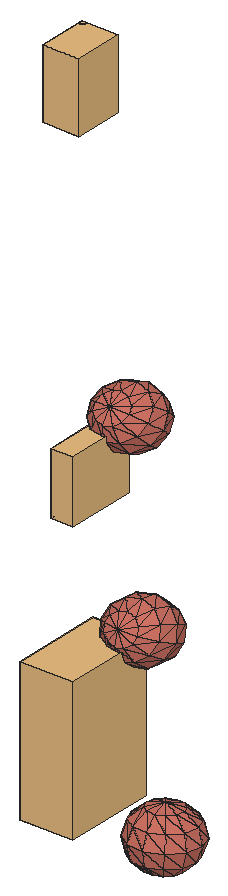
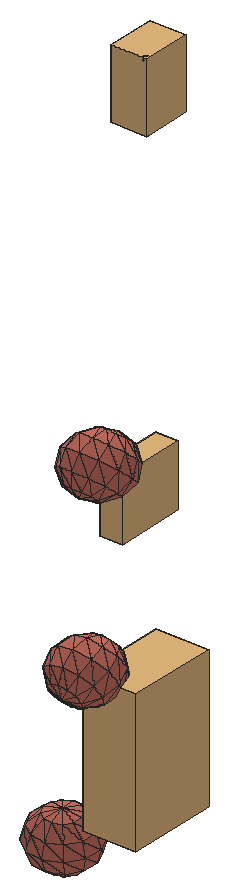
# SketchUp Ruby script. Lengths in inches.
U = 1.inch
M = Sketchup.active_model
def pt(a) = Geom::Point3d.new(a.map { |v| v * U })
def face(e, loops, mat)
  f = e.add_face(loops[0].map { |a| pt(a) })
  loops[1..].each { |l| e.add_face(l.map { |a| pt(a) }).erase! }
  f.material = f.back_material = mat if mat
  f
end
# faces: each face lists its corners as indices into pts; further lists are holes
def faces(e, pts, list, mat = nil) = list.each { |f| face(e, (f[0].is_a?(Array) ? f : [f]).map { |l| l.map { |i| pts[i] } }, mat) }
# xy, xz, yz: faces in a plane at the given z, y or x. An outline is a flat list of corners, or four numbers for a rectangle; further outlines are holes
def ring(l) = l.size == 4 ? [[l[0], l[1]], [l[2], l[1]], [l[2], l[3]], [l[0], l[3]]] : l.each_slice(2).to_a
def flat(e, list, mat, &to3) = list.each { |f| face(e, (f[0].is_a?(Array) ? f : [f]).map { |l| ring(l).map { |u, v| to3.(u, v) } }, mat) }
def xy(e, z, list, mat = nil) = flat(e, list, mat) { |x, y| [x, y, z] }
def xz(e, y, list, mat = nil) = flat(e, list, mat) { |x, z| [x, y, z] }
def yz(e, x, list, mat = nil) = flat(e, list, mat) { |y, z| [x, y, z] }
def lines(e, pts, list) = list.each { |a, b| e.add_line(pt(pts[a]), pt(pts[b])) }
# prism: a flat outline (further loops are holes) pulled along v
def prism(e, loops, v, mat = nil)
  f = face(e, loops, mat); d = Geom::Vector3d.new(v.map { |x| x * U })
  f.pushpull(f.normal.samedirection?(d) ? d.length : -d.length)
end
def box(e, o, s, mat = nil) = prism(e, [[o, [o[0] + s[0], o[1], o[2]], [o[0] + s[0], o[1] + s[1], o[2]], [o[0], o[1] + s[1], o[2]]]], [0, 0, s[2]], mat)
def at(x, y, z, deg = 0) = Geom::Transformation.translation(pt([x, y, z])) * Geom::Transformation.rotation(ORIGIN, Z_AXIS, deg.degrees)
def axes(o, x, y, z) = Geom::Transformation.new([*x, 0, *y, 0, *z, 0, *pt(o).to_a, 1])
def part(name) = M.definitions.add(name)
# library, detail: a bought-in or finely detailed component or shape, given as its bounding box
def library(name, o, s) = part(name).tap { |d| box(d.entities, o, s) }
def detail(e, o, s) = box(e.add_group.entities, o, s)
def put(e, d, t, mat = nil) = e.add_instance(d, t).tap { |i| i.material = mat if mat }
def group(e, t, mat = nil) = e.add_group.tap { |g| g.transformation = t; g.material = mat if mat }.entities
root = M.entities
M.materials.add("green").color = [174, 139, 102]
M.materials.add("vio").color = [206, 114, 100]
c1 = library("3DGeom~25_Defintion",[-351.97,-500,-258.4],[703.94,1000,516.8])
c2 = part("3DGeom~26_Defintion")
p = [[-344.73,487.39,-243.89],[-293.86,494.46,-251.4],[-311.18,491.2,-258.4],[-344.73,487.39,-243.89],[-311.18,491.2,-258.4],[-329.79,488.61,-255.65],
  [-344.73,487.39,-243.89],[-282.49,497.51,-236.53],[-293.86,494.46,-251.4],[-344.73,487.39,-243.89],[-351.97,487.85,-226.26],[-349.59,489.88,-207.5],
  [-344.73,487.39,-243.89],[-349.59,489.88,-207.5],[-338.22,492.93,-192.625],[-344.73,487.39,-243.89],[-280.11,499.54,-217.76],[-282.49,497.51,-236.53],
  [-344.73,487.39,-243.89],[-302.29,498.77,-188.375],[-287.36,500,-200.14],[-344.73,487.39,-243.89],[-287.36,500,-200.14],[-280.11,499.54,-217.76],
  [-344.73,487.39,-243.89],[-338.22,492.93,-192.625],[-320.91,496.1875,-185.625],[-344.73,487.39,-243.89],[-320.91,496.1875,-185.625],[-302.29,498.77,-188.375],
  [300.11,-500,207.2],[314.12,-496.86,194.8],[330.21,-489.05,190.33],[351.97,-468.47,207.5],[300.11,-500,207.2],[330.21,-489.05,190.33],
  [351.97,-468.47,207.5],[330.21,-489.05,190.33],[344.06,-478.66,194.98],[291.79,-490.37,241.23],[300.11,-500,207.2],[313.56,-469.79,258.4],
  [300.11,-500,207.2],[291.79,-490.37,241.23],[291.94,-497.625,224.19],[343.65,-458.84,241.54],[300.11,-500,207.2],[351.97,-468.47,207.5],
  [313.56,-469.79,258.4],[300.11,-500,207.2],[343.65,-458.84,241.54],[343.65,-458.84,241.54],[351.97,-468.47,207.5],[351.82,-461.21,224.54],
  [291.79,-490.37,241.23],[313.56,-469.79,258.4],[299.7,-480.18,253.76],[313.56,-469.79,258.4],[343.65,-458.84,241.54],[329.64,-461.98,253.93]]
faces(c2.entities,p,[[0,1,2],[3,4,5],[6,7,8],[9,10,11],[12,13,14],[15,16,17],[18,19,20],[21,22,23],
  [24,25,26],[27,28,29],[30,31,32],[33,34,35],[36,37,38],[39,40,41],[42,43,44],[45,46,47],
  [48,49,50],[51,52,53],[54,55,56],[57,58,59]],"green")
c3 = library("3DGeom~17_Defintion",[-322.12,-500,-186.09],[644.24,1000,372.18])
c4 = part("3DGeom~18_Defintion")
p = [[292.74,-500,-165.38],[307.55,-495.14,-174.52],[291.14,-497.07,-147.46],[307.55,-495.14,-174.52],[292.74,-500,-165.38],[299.25,-498.4,-172.01],
  [291.14,-497.07,-147.46],[307.55,-495.14,-174.52],[304.35,-489.29,-138.68],[304.35,-489.29,-138.68],[307.55,-495.14,-174.52],[319.15,-484.43,-147.83],
  [307.55,-495.14,-174.52],[315.42,-491.1,-172.22],[320.75,-487.36,-165.74],[320.75,-487.36,-165.74],[319.15,-484.43,-147.83],[320.75,-487.36,-165.74],
  [322.12,-484.92,-156.8125],[292.74,-500,-165.38],[291.14,-497.07,-147.46],[289.78,-499.51,-156.39],[304.35,-489.29,-138.68],[319.15,-484.43,-147.83],
  [312.65,-486.03,-141.19],[291.14,-497.07,-147.46],[304.35,-489.29,-138.68],[296.48,-493.33,-140.98],[-309.07,495.99,151.67],[-322.12,484.07,169.09],
  [-318.39,482.74,177.66],[-309.07,495.99,151.67],[-318.39,482.74,177.66],[-311.33,483.72,183.88],[-309.07,495.99,151.67],[-311.33,483.72,183.88],
  [-302.83,486.75,186.09],[-309.07,495.99,151.67],[-321.51,487.36,160.45],[-322.12,484.07,169.09],[-309.07,495.99,151.67],[-302.83,486.75,186.09],
  [-295.16,491.02,183.67],[-309.07,495.99,151.67],[-316.73,491.72,154.08],[-321.51,487.36,160.45],[-309.07,495.99,151.67],[-295.16,491.02,183.67],
  [-290.38,495.38,177.3],[-309.07,495.99,151.67],[-290.38,495.38,177.3],[-289.78,498.67,168.67],[-309.07,495.99,151.67],[-289.78,498.67,168.67],
  [-293.5,500,160.09],[-309.07,495.99,151.67],[-293.5,500,160.09],[-300.5625,499.02,153.87]]
faces(c4.entities,p,[[0,1,2],[3,4,5],[6,7,8],[9,10,11],[12,13,14],[11,10,15],[16,17,18],[19,20,21],
  [22,23,24],[25,26,27],[28,29,30],[31,32,33],[34,35,36],[37,38,39],[40,41,42],[43,44,45],
  [46,47,48],[49,50,51],[52,53,54],[55,56,57]],"green")
c5 = library("3DGeom~21_Defintion",[-500,-446.39,-160.99],[1000,892.78,321.97])
c6 = part("3DGeom~22_Defintion")
p = [[448.91,-442.9,-142.17],[471.3125,-423.55,-160.99],[450.7,-444.07,-105.16],[450.7,-444.07,-105.16],[471.3125,-423.55,-160.99],[474.89,-425.89,-86.96],
  [471.3125,-423.55,-160.99],[448.91,-442.9,-142.17],[458.1,-434.54,-155.85],[474.89,-425.89,-86.96],[471.3125,-423.55,-160.99],[497.29,-406.54,-105.77],
  [471.3125,-423.55,-160.99],[485,-412.87,-156.2],[495.5,-405.37,-142.78],[471.3125,-423.55,-160.99],[495.5,-405.37,-142.78],[495.5,-405.37,-142.78],
  [500,-403.05,-124.32],[448.91,-442.9,-142.17],[450.7,-444.07,-105.16],[446.2,-446.39,-123.62],[474.89,-425.89,-86.96],[488.1,-414.9,-92.09],
  [450.7,-444.07,-105.16],[474.89,-425.89,-86.96],[461.21,-436.57,-91.74],[-483.76,433.75,98.79],[-496.54,399.82,130.23],[-485.88,396.59,145.74],
  [-483.76,433.75,98.79],[-485.88,396.59,145.74],[-470.87,400.03,156.99],[-483.76,433.75,98.79],[-500,408.86,114.64],[-496.54,399.82,130.23],
  [-483.76,433.75,98.79],[-470.87,400.03,156.99],[-455.53,409.22,160.98],[-483.76,433.75,98.79],[-495.32,421.28,103.125],[-483.76,433.75,98.79],
  [-455.53,409.22,160.98],[-443.97,421.7,156.64],[-483.76,433.75,98.79],[-443.97,421.7,156.64],[-439.29,434.12,145.13],[-483.76,433.75,98.79],
  [-442.75,443.16,129.53],[-453.41,446.39,114.03],[-483.76,433.75,98.79],[-453.41,446.39,114.03],[-468.42,442.95,102.78],[-483.76,433.75,98.79],
  [-439.29,434.12,145.13],[-442.75,443.16,129.53]]
faces(c6.entities,p,[[0,1,2],[3,4,5],[6,7,8],[9,10,11],[12,13,14],[11,15,16],[11,17,18],[19,20,21],
  [22,11,23],[24,25,26],[27,28,29],[30,31,32],[33,34,35],[36,37,38],[39,40,34],[41,42,43],
  [44,45,46],[47,48,49],[50,51,52],[53,54,55]],"green")
c7 = part("3DGeom~225_Defintion")
p = [[77.58,-12.43,-500],[-128.33,-244.69,-395.82],[-181.28,-36.33,-470.68],[95.84,-224,-421.21],[315.65,14.8,-395.34],[38.53,202.47,-444.81],
  [244.7,226.05,-354.18],[-310.44,-256.96,-261.21],[-391.56,-50.49,-315.24],[-310.44,-256.96,-261.21],[-185.65,181.77,-419.42],[-391.56,-50.49,-315.24],
  [-10.85,363.12,-270.44],[108.1875,376.73,-218.11],[-10.85,363.12,-270.44],[108.1875,376.73,-218.11],[-41,-387.49,-214.9],[88.43,-375.54,-229.56],
  [-41,-387.49,-214.9],[302.01,-200.41,-330.58],[-391.56,-50.49,-315.24],[-367.76,169.5,-284.8125],[-140.27,351.16,-255.78],[-367.76,169.5,-284.8125],
  [-10.85,363.12,-270.44],[-140.27,351.16,-255.78],[-128.33,-244.69,-395.82],[-146.14,-394.58,-137.18],[-310.44,-256.96,-261.21],[-128.33,-244.69,-395.82],
  [-41,-387.49,-214.9],[469.13,38.07,-184.76],[302.01,-200.41,-330.58],[315.65,14.8,-395.34],[377.625,246.2,-171.81],[315.65,14.8,-395.34],
  [244.7,226.05,-354.18],[377.625,246.2,-171.81],[315.65,14.8,-395.34],[184.93,388.36,-112.82],[244.7,226.05,-354.18],[108.1875,376.73,-218.11],
  [377.625,246.2,-171.81],[244.7,226.05,-354.18],[207.46,-361.93,-177.23],[434.94,-180.27,-148.2],[207.46,-361.93,-177.23],[302.01,-200.41,-330.58],
  [302.01,-200.41,-330.58],[-391.56,-50.49,-315.24],[-401.6875,-257.51,-53.44],[-496.92,-51.13,-75.34],[-310.44,-256.96,-261.21],[-367.76,169.5,-284.8125],
  [-459,168.95,-77.05],[-245.41,344.08,-178.0625],[-140.27,351.16,-255.78],[-367.76,169.5,-284.8125],[-245.41,344.08,-178.0625],[-10.85,363.12,-270.44],
  [-140.27,351.16,-255.78],[-57.32,426.47,-23.6],[-310.44,-256.96,-261.21],[-198.82,-394.9,-17.23],[-401.6875,-257.51,-53.44],[-310.44,-256.96,-261.21],
  [-245.41,344.08,-178.0625],[88.43,-375.54,-229.56],[57.32,-426.47,23.6],[88.43,-375.54,-229.56],[207.46,-361.93,-177.23],[496.92,51.13,75.34],
  [401.6875,257.51,53.44],[377.625,246.2,-171.81],[401.6875,257.51,53.44],[-245.41,344.08,-178.0625],[-298.1,343.77,-58.11],[-298.1,343.77,-58.11],
  [207.46,-361.93,-177.23],[284.2,-350.3,-71.9375],[284.2,-350.3,-71.9375],[207.46,-361.93,-177.23],[198.82,394.9,17.23],[401.6875,257.51,53.44],
  [459,-168.95,77.05],[-469.13,-38.07,184.76],[-434.94,180.27,148.2],[-298.1,343.77,-58.11],[-377.625,-246.2,171.81],[284.2,-350.3,-71.9375],
  [298.1,-343.77,58.11],[298.1,-343.77,58.11],[-298.1,343.77,-58.11],[-284.2,350.3,71.9375],[-284.2,350.3,71.9375],[-401.6875,-257.51,-53.44],
  [-184.93,-388.36,112.82],[-401.6875,-257.51,-53.44],[-377.625,-246.2,171.81],[-207.46,361.93,177.23],[-88.43,375.54,229.56],[41,387.49,214.9],
  [146.14,394.58,137.18],[-108.1875,-376.73,218.11],[10.85,-363.12,270.44],[-108.1875,-376.73,218.11],[140.27,-351.16,255.78],[10.85,-363.12,270.44],
  [298.1,-343.77,58.11],[245.41,-344.08,178.0625],[245.41,-344.08,178.0625],[140.27,-351.16,255.78],[310.44,256.96,261.21],[401.6875,257.51,53.44],
  [310.44,256.96,261.21],[367.76,-169.5,284.8125],[245.41,-344.08,178.0625],[-284.2,350.3,71.9375],[-302.01,200.41,330.58],[-284.2,350.3,71.9375],
  [-302.01,200.41,330.58],[-207.46,361.93,177.23],[391.56,50.49,315.24],[310.44,256.96,261.21],[-377.625,-246.2,171.81],[-108.1875,-376.73,218.11],
  [-315.65,-14.8,395.34],[-315.65,-14.8,395.34],[-302.01,200.41,330.58],[-377.625,-246.2,171.81],[-108.1875,-376.73,218.11],[-244.7,-226.05,354.18],
  [-244.7,-226.05,354.18],[-207.46,361.93,177.23],[-302.01,200.41,330.58],[-95.84,224,421.21],[-207.46,361.93,177.23],[-88.43,375.54,229.56],
  [185.65,-181.77,419.42],[140.27,-351.16,255.78],[245.41,-344.08,178.0625],[245.41,-344.08,178.0625],[367.76,-169.5,284.8125],[-244.7,-226.05,354.18],
  [-315.65,-14.8,395.34],[-88.43,375.54,229.56],[128.33,244.69,395.82],[41,387.49,214.9],[128.33,244.69,395.82],[-244.7,-226.05,354.18],
  [-108.1875,-376.73,218.11],[10.85,-363.12,270.44],[-88.43,375.54,229.56],[128.33,244.69,395.82],[-38.53,-202.47,444.81],[128.33,244.69,395.82],
  [391.56,50.49,315.24],[310.44,256.96,261.21],[181.28,36.33,470.68],[367.76,-169.5,284.8125],[367.76,-169.5,284.8125],[391.56,50.49,315.24],
  [128.33,244.69,395.82],[391.56,50.49,315.24],[-315.65,-14.8,395.34],[-77.58,12.43,500],[128.33,244.69,395.82]]
faces(c7.entities,p,[[0,1,2],[0,3,1],[4,3,0],[5,0,2],[6,0,5],[6,4,0],[2,7,8],[2,1,9],
  [10,2,11],[5,2,10],[12,5,10],[13,5,14],[15,6,5],[3,16,1],[3,17,18],[19,17,3],
  [4,19,3],[10,20,21],[22,10,23],[24,10,25],[26,27,28],[29,30,27],[31,32,33],[34,35,36],
  [37,31,38],[39,40,41],[39,42,43],[19,44,17],[45,46,47],[31,45,48],[49,50,51],[49,52,50],
  [53,49,51],[53,51,54],[55,53,54],[56,57,58],[59,60,61],[41,59,61],[62,63,64],[65,27,63],
  [60,66,61],[30,67,68],[69,70,68],[39,41,61],[27,30,68],[71,45,31],[72,31,73],[74,71,31],
  [75,54,76],[66,77,61],[78,79,68],[45,80,81],[82,42,39],[82,83,42],[84,80,45],[71,84,45],
  [63,27,68],[82,39,61],[54,51,85],[54,85,86],[87,54,86],[51,50,88],[51,88,85],[89,90,68],
  [84,91,80],[92,86,93],[77,94,61],[95,63,96],[97,96,98],[94,99,61],[99,100,61],[100,101,61],
  [101,102,61],[102,82,61],[96,63,68],[102,83,82],[103,96,68],[104,105,68],[106,107,68],[108,109,68],
  [110,111,68],[112,71,113],[102,114,83],[115,116,91],[115,91,84],[117,86,118],[119,120,121],[122,84,71],
  [123,122,71],[122,115,84],[124,96,125],[101,114,102],[86,85,126],[86,127,128],[129,130,131],[85,88,132],
  [133,134,135],[136,135,137],[138,139,140],[138,141,142],[85,143,144],[145,146,147],[101,148,114],[149,150,151],
  [152,135,153],[154,151,139],[154,139,138],[155,156,157],[149,151,154],[158,138,159],[158,160,161],[162,158,163],
  [134,164,165],[134,165,135],[164,149,154],[164,154,165],[135,158,166],[165,154,138],[165,138,158],[135,165,158]],"vio")
c8 = part("3DGeom~195_Defintion")
p = [[166.45,-153.95,-435.25],[-186.98,-146.09,-430.65],[-6.51,0,-500],[325.5,12.77,-379.3],[-335.26,-12.77,-370.7],[-177.72,153.95,-430.77],
  [175.71,146.09,-435.37],[397.32,176.07,-221.71],[27.43,279.42,-375.42],[310.84,253.04,-254.09],[27.43,279.42,-375.42],[397.32,176.07,-221.71],
  [310.84,253.04,-254.09],[-37.19,-279.42,-374.58],[294.8125,-266.65,-253.88],[436.66,-84.83,-222.23],[436.66,-84.83,-222.23],[-442.29,84.83,-210.79],
  [-442.29,84.83,-210.79],[-301.32,266.65,-246.12],[27.43,279.42,-375.42],[-301.32,266.65,-246.12],[-317.35,-253.04,-245.91],[-402.96,-176.07,-211.3],
  [-402.96,-176.07,-211.3],[461.5,119.72,-131.03],[436.66,-84.83,-222.23],[325.5,12.77,-379.3],[325.5,12.77,-379.3],[397.32,176.07,-221.71],
  [310.84,253.04,-254.09],[27.43,279.42,-375.42],[225.23,330.02,-219.47],[27.43,279.42,-375.42],[-301.32,266.65,-246.12],[-79.61,377.03,-215.51],
  [225.23,330.02,-219.47],[27.43,279.42,-375.42],[-79.61,377.03,-215.51],[73.97,-377.02,-217.51],[-230.87,-330.02,-213.54],[-37.19,-279.42,-374.58],
  [73.97,-377.02,-217.51],[-230.87,-330.02,-213.54],[-335.26,-12.77,-370.7],[-402.96,-176.07,-211.3],[-464.76,-119.72,-118.97],[-335.26,-12.77,-370.7],
  [-442.29,84.83,-210.79],[310.84,253.04,-254.09],[362.6875,292.19,-4.72],[225.23,330.02,-219.47],[344.18,-307.91,-4.48],[73.97,-377.02,-217.51],
  [294.8125,-266.65,-253.88],[479.41,-120.56,-6.24],[344.18,-307.91,-4.48],[294.8125,-266.65,-253.88],[294.8125,-266.65,-253.88],[-301.32,266.65,-246.12],
  [-479.41,120.56,6.24],[-301.32,266.65,-246.12],[-344.18,307.91,4.48],[-301.32,266.65,-246.12],[-344.18,307.91,4.48],[-317.35,-253.04,-245.91],
  [-230.87,-330.02,-213.54],[-362.6875,-292.19,4.72],[-317.35,-253.04,-245.91],[-362.6875,-292.19,4.72],[486.1875,99.09,-6.33],[163.4375,386.37,-127.15],
  [362.6875,292.19,-4.72],[116.72,-412.75,-1.52],[-166.69,-386.37,-122.85],[73.97,-377.02,-217.51],[344.18,-307.91,-4.48],[73.97,-377.02,-217.51],
  [73.97,-377.02,-217.51],[-230.87,-330.02,-213.54],[-116.72,412.75,1.52],[-230.87,-330.02,-213.54],[-362.6875,-292.19,4.72],[-362.6875,-292.19,4.72],
  [-486.1875,-99.09,6.33],[142.01,407,-1.85],[362.6875,292.19,-4.72],[-142.01,-407,1.85],[-362.6875,-292.19,4.72],[464.76,119.72,118.97],
  [442.29,-84.83,210.79],[402.96,176.07,211.3],[317.35,253.04,245.91],[230.87,330.02,213.54],[166.69,386.37,122.85],[362.6875,292.19,-4.72],
  [230.87,330.02,213.54],[362.6875,292.19,-4.72],[301.32,-266.65,246.12],[344.18,-307.91,-4.48],[301.32,-266.65,246.12],[-73.97,377.02,217.51],
  [79.61,-377.03,215.51],[301.32,-266.65,246.12],[-294.8125,266.65,253.88],[-294.8125,266.65,253.88],[-163.4375,-386.37,127.15],[-344.18,307.91,4.48],
  [-436.66,84.83,222.23],[-344.18,307.91,4.48],[-436.66,84.83,222.23],[-294.8125,266.65,253.88],[-225.24,-330.02,219.47],[-225.24,-330.02,219.47],
  [-310.84,-253.04,254.09],[-362.6875,-292.19,4.72],[-461.5,-119.72,131.03],[-362.6875,-292.19,4.72],[-397.32,-176.07,221.71],[-362.6875,-292.19,4.72],
  [-310.84,-253.04,254.09],[-397.32,-176.07,221.71],[-362.6875,-292.19,4.72],[-436.66,84.83,222.23],[37.19,279.42,374.58],[37.19,279.42,374.58],
  [230.87,330.02,213.54],[-27.43,-279.42,375.42],[-27.43,-279.42,375.42],[-436.66,84.83,222.23],[-397.32,-176.07,221.71],[335.26,12.77,370.7],
  [301.32,-266.65,246.12],[442.29,-84.83,210.79],[335.26,12.77,370.7],[317.35,253.04,245.91],[335.26,12.77,370.7],[402.96,176.07,211.3],
  [230.87,330.02,213.54],[37.19,279.42,374.58],[186.98,146.09,430.65],[230.87,330.02,213.54],[317.35,253.04,245.91],[177.72,-153.95,430.77],
  [-27.43,-279.42,375.42],[79.61,-377.03,215.51],[79.61,-377.03,215.51],[301.32,-266.65,246.12],[-73.97,377.02,217.51],[-294.8125,266.65,253.88],
  [-166.45,153.95,435.25],[-73.97,377.02,217.51],[-175.71,-146.09,435.37],[-310.84,-253.04,254.09],[-225.24,-330.02,219.47],[-225.24,-330.02,219.47],
  [-325.5,-12.77,379.3],[-397.32,-176.07,221.71],[-436.66,84.83,222.23],[-397.32,-176.07,221.71],[-325.5,-12.77,379.3],[-436.66,84.83,222.23],
  [317.35,253.04,245.91],[335.26,12.77,370.7],[335.26,12.77,370.7],[301.32,-266.65,246.12],[335.26,12.77,370.7],[6.51,0,500]]
faces(c8.entities,p,[[0,1,2],[3,0,2],[2,1,4],[2,4,5],[6,2,5],[3,2,6],[7,3,6],[6,5,8],
  [9,6,10],[11,6,12],[0,13,1],[14,13,0],[15,14,0],[16,0,3],[5,4,17],[5,18,19],
  [20,5,21],[13,22,1],[1,22,23],[1,24,4],[25,26,27],[25,28,29],[30,31,32],[33,34,35],
  [36,37,38],[39,40,41],[14,42,13],[13,43,22],[44,45,46],[47,46,48],[29,49,50],[49,51,50],
  [52,53,54],[55,56,57],[55,58,26],[59,48,60],[61,60,62],[38,63,64],[65,66,67],[45,68,69],
  [70,55,26],[70,26,25],[25,29,50],[36,71,72],[36,38,71],[73,74,75],[76,73,77],[78,74,79],
  [38,64,80],[71,38,80],[81,74,82],[46,45,83],[48,46,84],[48,84,60],[70,25,50],[71,85,86],
  [71,80,85],[73,87,74],[74,87,82],[84,46,88],[89,55,70],[89,70,50],[90,56,55],[89,90,55],
  [91,89,50],[92,91,50],[93,92,50],[85,94,95],[94,96,97],[98,73,99],[90,100,56],[85,80,101],
  [85,101,94],[102,87,73],[103,102,73],[80,64,104],[80,105,101],[87,106,82],[102,106,87],[107,60,108],
  [109,110,111],[106,112,82],[113,114,115],[116,84,117],[118,116,119],[120,121,122],[60,84,116],[60,116,123],
  [91,90,89],[94,101,124],[94,125,126],[127,112,106],[128,106,102],[129,116,130],[131,132,133],[91,134,90],
  [135,136,137],[138,139,140],[141,140,142],[143,144,145],[143,146,147],[148,149,150],[151,150,139],[152,153,154],
  [152,155,144],[156,157,153],[158,159,160],[149,161,156],[162,140,163],[164,143,165],[149,156,150],[156,153,152],
  [140,143,166],[139,150,167],[139,167,140],[167,152,144],[167,144,143],[150,156,152],[140,167,143],[150,152,167]],"vio")
c9 = part("3DGeom~193_Defintion")
p = [[111.73,-187.4,-434.54],[-226.37,-99.64,-430.14],[-6.51,0,-500],[317.5,-62.65,-379.2],[-327.26,62.65,-370.81],[215.1,99.64,-435.89],
  [-123,187.4,-431.49],[438.19,78.88,-222.25],[438.19,78.88,-222.25],[379.08,172.58,-254.98],[114.21,261.93,-376.55],[379.08,172.58,-254.98],
  [114.21,261.93,-376.55],[200.03,-324.58,-252.65],[-123.97,-261.93,-373.45],[393.97,-181.45,-221.67],[393.97,-181.45,-221.67],[-399.61,181.45,-211.34],
  [-399.61,181.45,-211.34],[-206.54,324.58,-247.35],[114.21,261.93,-376.55],[-206.54,324.58,-247.35],[-385.58,-172.58,-245.02],[-226.37,-99.64,-430.14],
  [-385.58,-172.58,-245.02],[-443.83,-78.88,-210.77],[-226.37,-99.64,-430.14],[-327.26,62.65,-370.81],[482.35,10.29,-131.3],[393.97,-181.45,-221.67],
  [317.5,-62.65,-379.2],[317.5,-62.65,-379.2],[438.19,78.88,-222.25],[379.08,172.58,-254.98],[114.21,261.93,-376.55],[320.83,266.28,-220.72],
  [114.21,261.93,-376.55],[-206.54,324.58,-247.35],[41.87,380.73,-217.09],[320.83,266.28,-220.72],[114.21,261.93,-376.55],[41.87,380.73,-217.09],
  [-47.5,-380.73,-215.93],[-326.46,-266.28,-212.3],[-123.97,-261.93,-373.45],[-47.5,-380.73,-215.93],[-326.46,-266.28,-212.3],[-385.58,-172.58,-245.02],
  [-327.26,62.65,-370.81],[-485.6,-10.29,-118.7],[-327.26,62.65,-370.81],[-399.61,181.45,-211.34],[379.08,172.58,-254.98],[441.47,199.28,-5.74],
  [320.83,266.28,-220.72],[234.74,-374.79,-3.05],[-47.5,-380.73,-215.93],[200.03,-324.58,-252.65],[424.02,-224.9375,-5.52],[234.74,-374.79,-3.05],
  [200.03,-324.58,-252.65],[200.03,-324.58,-252.65],[-206.54,324.58,-247.35],[-424.02,224.9375,5.52],[-206.54,324.58,-247.35],[-234.74,374.79,3.05],
  [-206.54,324.58,-247.35],[-234.74,374.79,3.05],[-326.46,-266.28,-212.3],[-441.47,-199.28,5.74],[499.7,-14.8125,-6.5],[279.06,334.87,-128.65],
  [320.83,266.28,-220.72],[279.06,334.87,-128.65],[279.06,334.87,-128.65],[17.45,424.22,-0.23],[-17.45,-424.22,0.23],[-282.3125,-334.87,-121.35],
  [-47.5,-380.73,-215.93],[234.74,-374.79,-3.05],[-47.5,-380.73,-215.93],[-47.5,-380.73,-215.93],[-326.46,-266.28,-212.3],[-326.46,-266.28,-212.3],
  [-282.3125,-334.87,-121.35],[-499.7,14.8125,6.5],[264.96,359.98,-3.45],[279.06,334.87,-128.65],[264.96,359.98,-3.45],[-264.96,-359.98,3.45],
  [-282.3125,-334.87,-121.35],[-264.96,-359.98,3.45],[485.6,10.29,118.7],[443.83,78.88,210.77],[385.58,172.58,245.02],[326.46,266.28,212.3],
  [282.3125,334.87,121.35],[399.61,-181.45,211.34],[264.96,359.98,-3.45],[47.5,380.73,215.93],[282.3125,334.87,121.35],[264.96,359.98,-3.45],
  [206.54,-324.58,247.36],[234.74,-374.79,-3.05],[206.54,-324.58,247.36],[-200.03,324.58,252.65],[-200.03,324.58,252.65],[-41.87,-380.73,217.09],
  [206.54,-324.58,247.36],[-234.74,374.79,3.05],[-393.97,181.45,221.67],[-234.74,374.79,3.05],[-393.97,181.45,221.67],[-200.03,324.58,252.65],
  [-279.06,-334.87,128.65],[-264.96,-359.98,3.45],[-279.06,-334.87,128.65],[-482.35,-10.29,131.3],[-393.97,181.45,221.67],[-279.06,-334.87,128.65],
  [-320.83,-266.28,220.72],[-320.83,-266.28,220.72],[-379.08,-172.58,254.98],[-438.19,-78.88,222.25],[-379.08,-172.58,254.98],[-438.19,-78.88,222.25],
  [282.3125,334.87,121.35],[123.97,261.93,373.45],[282.3125,334.87,121.35],[123.97,261.93,373.45],[326.46,266.28,212.3],[-114.21,-261.93,376.55],
  [-114.21,-261.93,376.55],[-320.83,-266.28,220.72],[-393.97,181.45,221.67],[-438.19,-78.88,222.25],[327.26,-62.65,370.81],[327.26,-62.65,370.81],
  [206.54,-324.58,247.36],[399.61,-181.45,211.34],[326.46,266.28,212.3],[123.97,261.93,373.45],[226.37,99.64,430.14],[326.46,266.28,212.3],
  [226.37,99.64,430.14],[385.58,172.58,245.02],[47.5,380.73,215.93],[-200.03,324.58,252.65],[-111.73,187.4,434.54],[47.5,380.73,215.93],
  [123,-187.4,431.49],[-114.21,-261.93,376.55],[-41.87,-380.73,217.09],[-41.87,-380.73,217.09],[206.54,-324.58,247.36],[-215.1,-99.64,435.89],
  [-379.08,-172.58,254.98],[-320.83,-266.28,220.72],[-320.83,-266.28,220.72],[-393.97,181.45,221.67],[-438.19,-78.88,222.25],[-317.5,62.65,379.2],
  [-393.97,181.45,221.67],[-317.5,62.65,379.2],[-438.19,-78.88,222.25],[226.37,99.64,430.14],[327.26,-62.65,370.81],[206.54,-324.58,247.36],
  [226.37,99.64,430.14],[327.26,-62.65,370.81],[6.51,0,500],[226.37,99.64,430.14],[226.37,99.64,430.14]]
faces(c9.entities,p,[[0,1,2],[3,0,2],[2,1,4],[3,2,5],[2,4,6],[5,2,6],[7,3,5],[8,5,9],
  [5,6,10],[11,5,12],[13,14,0],[15,13,0],[0,14,1],[16,0,3],[6,4,17],[6,18,19],
  [20,6,21],[14,22,1],[23,24,25],[26,25,27],[28,29,30],[28,31,32],[33,34,35],[36,37,38],
  [39,40,41],[42,43,44],[13,45,14],[14,46,47],[48,25,49],[50,49,51],[32,52,53],[52,54,53],
  [55,56,57],[58,59,60],[58,61,29],[62,51,63],[64,63,65],[41,66,67],[24,68,69],[25,24,69],
  [28,32,53],[70,58,29],[70,29,28],[54,71,53],[72,41,73],[74,41,75],[41,67,75],[76,77,78],
  [79,76,80],[81,77,82],[83,84,69],[51,49,85],[51,85,63],[49,25,69],[70,28,53],[71,86,53],
  [87,75,88],[76,89,77],[90,91,69],[85,49,69],[92,58,70],[92,70,53],[93,92,53],[94,93,53],
  [95,94,53],[86,96,53],[96,95,53],[97,59,58],[92,97,58],[98,99,100],[101,75,99],[102,76,103],
  [97,104,59],[75,67,105],[75,106,99],[107,89,76],[108,107,76],[109,63,110],[111,112,113],[107,114,89],
  [115,116,69],[63,85,117],[63,117,118],[119,120,69],[121,122,69],[117,85,69],[123,117,69],[124,125,69],
  [93,97,92],[126,99,127],[128,129,130],[131,114,107],[132,133,114],[134,117,135],[93,136,97],[94,136,93],
  [137,138,139],[140,141,142],[143,144,145],[146,147,148],[149,148,141],[150,151,152],[150,153,154],[155,156,157],
  [155,158,151],[159,160,161],[147,162,163],[163,164,156],[94,165,136],[166,150,167],[147,163,148],[163,156,155],
  [168,150,169],[141,148,170],[141,170,171],[170,155,151],[170,151,150],[148,163,155],[172,170,150],[148,155,170]],"vio")
g1 = group(root,at(15.3125,38.42,26.21))
put(g1,c1,axes([3.34,0.21,15.8],[0,0.0004,0],[0,0,-0.0004],[-0.0004,0,0]),"green")
put(g1,c2,axes([3.34,0.21,15.8],[0,0.0004,0],[0,0,-0.0004],[-0.0004,0,0]),"green")
g2 = group(root,at(15.3125,38.42,26.21))
put(g2,c3,axes([3.3125,0.26,12.43],[0,0.00081,0],[0,0,-0.00081],[-0.00081,0,0]),"green")
put(g2,c4,axes([3.3125,0.26,12.43],[0,0.00081,0],[0,0,-0.00081],[-0.00081,0,0]),"green")
g3 = group(root,at(15.3125,38.42,26.21))
put(g3,c5,axes([3.32,0.3,13.74],[0,0.0004,0],[0,0,-0.0004],[-0.0004,0,0]),"green")
put(g3,c6,axes([3.32,0.3,13.74],[0,0.0004,0],[0,0,-0.0004],[-0.0004,0,0]),"green")
g4 = group(root,at(15.3125,38.42,26.21))
put(g4,c7,axes([3.63,0.45,11.9],[0,0.00039,0],[0,0,-0.00039],[-0.00039,0,0]),"vio")
g5 = group(root,at(15.3125,38.42,26.21))
put(g5,c8,axes([3.375,0.52,13.9375],[0,0.00039,0],[0,0,-0.00039],[-0.00039,0,0]),"vio")
g6 = group(root,at(15.3125,38.42,26.21))
put(g6,c9,axes([3.44,0.53,12.86],[0,0.00039,0],[0,0,-0.00039],[-0.00039,0,0]),"vio")
